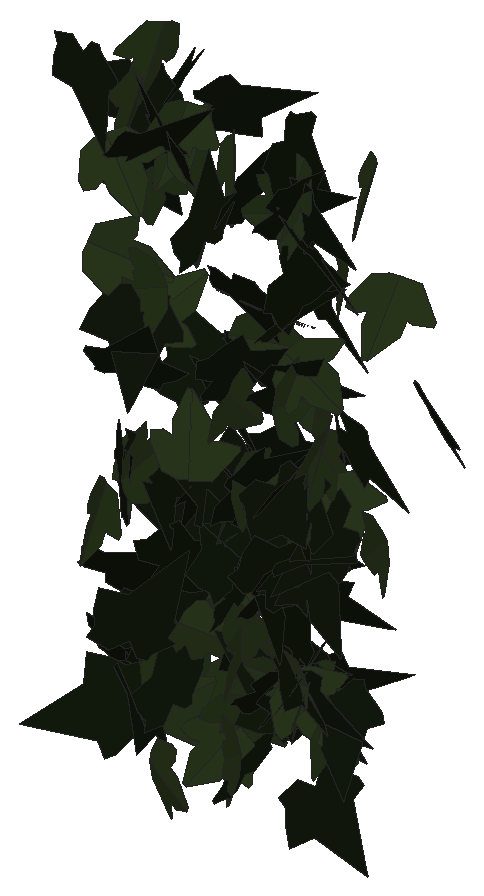
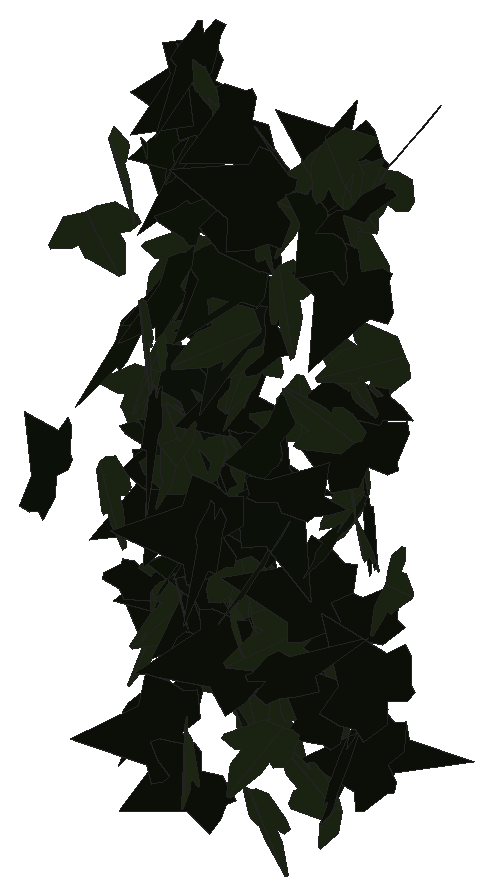
# SketchUp Ruby script. Lengths in inches.
U = 1.inch
M = Sketchup.active_model
def pt(a) = Geom::Point3d.new(a.map { |v| v * U })
def face(e, loops, mat)
  f = e.add_face(loops[0].map { |a| pt(a) })
  loops[1..].each { |l| e.add_face(l.map { |a| pt(a) }).erase! }
  f.material = f.back_material = mat if mat
  f
end
# faces: each face lists its corners as indices into pts; further lists are holes
def faces(e, pts, list, mat = nil) = list.each { |f| face(e, (f[0].is_a?(Array) ? f : [f]).map { |l| l.map { |i| pts[i] } }, mat) }
# xy, xz, yz: faces in a plane at the given z, y or x. An outline is a flat list of corners, or four numbers for a rectangle; further outlines are holes
def ring(l) = l.size == 4 ? [[l[0], l[1]], [l[2], l[1]], [l[2], l[3]], [l[0], l[3]]] : l.each_slice(2).to_a
def flat(e, list, mat, &to3) = list.each { |f| face(e, (f[0].is_a?(Array) ? f : [f]).map { |l| ring(l).map { |u, v| to3.(u, v) } }, mat) }
def xy(e, z, list, mat = nil) = flat(e, list, mat) { |x, y| [x, y, z] }
def xz(e, y, list, mat = nil) = flat(e, list, mat) { |x, z| [x, y, z] }
def yz(e, x, list, mat = nil) = flat(e, list, mat) { |y, z| [x, y, z] }
def lines(e, pts, list) = list.each { |a, b| e.add_line(pt(pts[a]), pt(pts[b])) }
# prism: a flat outline (further loops are holes) pulled along v
def prism(e, loops, v, mat = nil)
  f = face(e, loops, mat); d = Geom::Vector3d.new(v.map { |x| x * U })
  f.pushpull(f.normal.samedirection?(d) ? d.length : -d.length)
end
def box(e, o, s, mat = nil) = prism(e, [[o, [o[0] + s[0], o[1], o[2]], [o[0] + s[0], o[1] + s[1], o[2]], [o[0], o[1] + s[1], o[2]]]], [0, 0, s[2]], mat)
def at(x, y, z, deg = 0) = Geom::Transformation.translation(pt([x, y, z])) * Geom::Transformation.rotation(ORIGIN, Z_AXIS, deg.degrees)
def axes(o, x, y, z) = Geom::Transformation.new([*x, 0, *y, 0, *z, 0, *pt(o).to_a, 1])
def part(name) = M.definitions.add(name)
# library, detail: a bought-in or finely detailed component or shape, given as its bounding box
def library(name, o, s) = part(name).tap { |d| box(d.entities, o, s) }
def detail(e, o, s) = box(e.add_group.entities, o, s)
def put(e, d, t, mat = nil) = e.add_instance(d, t).tap { |i| i.material = mat if mat }
def group(e, t, mat = nil) = e.add_group.tap { |g| g.transformation = t; g.material = mat if mat }.entities
root = M.entities
M.materials.add("efeu1").color = [18, 25, 13]
M.materials.add("efeu2").color = [43, 57, 29]
c1 = part("ivyleaf_9")
p = [[1.54,2.16,1.25],[1.36,2.04,1.19],[-0.21,0.99,0.68],[-0.71,1.11,0.82],[-0.85,0.86,0.67],[-0.8,0.17,0.21],
  [-0.9,-0.01,0.1],[-0.67,-0.16,-0.02],[-0.08,-0.08,-0.05],[-0.03,-0.6,-0.4],[0.65,-0.88,-0.66],[0.83,-0.6,-0.49],
  [1.29,-0.42,-0.43],[1.8125,-0.07,-0.26],[1.21,0.44,0.15]]
faces(c1.entities,p,[[0,1,2,3,4,5,6,7,8,9,10,11,12,13,14]],"efeu1")
c2 = part("ivyleaf_10")
p = [[0,0.5,-0.03],[-0.0625,2.02,-0.43],[-0.19,2.01,-0.46],[-0.54,1.05,-0.29],[-0.52,0.625,-0.18],[-0.83,0.76,-0.28],
  [-1.16,0.64,-0.33],[-1.15,0.33,-0.24],[-0.77,-0.39,0.02],[-0.3,-0.51,0.16],[0.04,-0.48,0.23],[-0.02,2.01,-0.4375],
  [-0.06,2.01,-0.43],[0.04,-0.49,0.23],[0.67,-0.49,0.14],[1.38,0.36,-0.2],[1.375,0.51,-0.24],[0.81,0.65,-0.19],
  [0.62,0.59,-0.15],[0.6,1.09,-0.28],[0.5,1.23,-0.31]]
faces(c2.entities,p,[[0,1,2,3,4,5,6,7,8,9,10],[11,12,0,13,14,15,16,17,18,19,20]],"efeu2")
put(root,c1,axes([42.93,222.36,233.58],[0.15488,-0.47136,0.06189],[0.02451,-0.05709,-0.49613],[0.47478,0.15671,0.00543]))
put(root,c2,axes([43.24,222.41,226.64],[-0.02488,0.30941,-0.39197],[0.00458,-0.3923,-0.30996],[-0.49936,-0.01901,0.01669]))
put(root,c1,axes([42.96,222.87,225.19],[0.44169,0.18488,-0.14397],[0.13357,0.05377,0.47882],[0.19253,-0.46144,-0.00189]))
put(root,c1,axes([43.4375,223.5,232.54],[0.09096,0.30125,0.38855],[-0.03285,0.39799,-0.30088],[-0.49056,0.02921,0.09219]))
put(root,c2,axes([43.01,222.72,230.36],[0.11872,0.11072,0.47291],[0.33753,0.33126,-0.16229],[-0.34925,0.35778,0.00392]))
put(root,c1,axes([43.19,223.3,232.87],[0.01893,-0.49026,-0.09637],[-0.01328,0.09592,-0.49053],[0.49947,0.02113,-0.00939]))
put(root,c1,axes([43.28,223.01,231.71],[0.38774,0.31259,-0.04407],[-0.03007,-0.03292,-0.49801],[-0.31425,0.38885,-0.00673]))
put(root,c1,axes([43.27,223.64,223.89],[-0.00944,-0.14367,0.47882],[-0.06893,-0.47396,-0.14357],[0.49514,-0.06872,-0.01086]))
put(root,c2,axes([43.33,223.01,232.89],[0.08318,-0.37439,0.32079],[0.16253,-0.28632,-0.3763],[0.46547,0.16688,0.07406]))
put(root,c1,axes([43.01,222.79,224.13],[0.36576,-0.15936,0.30137],[0.27375,-0.12612,-0.39894],[0.20317,0.45683,-0.00501]))
put(root,c2,axes([43.44,223.34,233.63],[-0.07219,-0.46219,0.17654],[0.05138,-0.18445,-0.46189],[0.49209,-0.04854,0.07413]))
put(root,c1,axes([43.84,222.13,223.7],[-0.32895,-0.11375,0.35896],[-0.34056,-0.11349,-0.34805],[0.16066,-0.47348,-0.00281]))
put(root,c2,axes([43.85,222.74,230.08],[0.20662,-0.13869,-0.43368],[-0.37197,0.22324,-0.24861],[0.26258,0.42536,-0.01093]))
put(root,c1,axes([43.4,222.69,228.625],[0.47942,0.12712,0.06323],[-0.0611,-0.01628,0.49599],[0.12816,-0.4833,-0.00007]))
put(root,c2,axes([43.72,222.75,231.92],[-0.48355,-0.11831,0.04669],[-0.04423,-0.01567,-0.49779],[0.11925,-0.48555,0.00469]))
put(root,c1,axes([43.6,222.77,229.65],[-0.33168,-0.29939,-0.22441],[0.16944,0.14719,-0.4468],[0.33359,-0.37243,0.00381]))
put(root,c1,axes([43.97,224.05,225.63],[-0.18764,-0.4073,-0.22113],[-0.07372,-0.2093,0.44806],[-0.45755,0.20075,0.0185]))
put(root,c2,axes([43.44,223.21,229.27],[0.35959,0.00728,-0.34733],[0.33553,0.12232,0.34994],[0.09006,-0.48475,0.08308]))
put(root,c1,axes([44.03,223.76,228.27],[-0.45268,-0.21087,-0.0249],[-0.02211,-0.0115,0.49938],[-0.21118,0.45321,0.00109]))
put(root,c1,axes([43.59,222.35,227.02],[-0.04067,0.11489,0.48492],[0.10552,-0.47351,0.12104],[0.48704,0.11218,0.01426]))
put(root,c2,axes([43.62,222.55,227.51],[0.346,-0.22098,0.2854],[0.23724,-0.15873,-0.41052],[0.27204,0.41949,-0.00499]))
put(root,c2,axes([43.71,224.36,224.9375],[0.14333,0.38801,0.2809],[0.1107,0.25843,-0.41347],[-0.46605,0.18072,-0.01182]))
put(root,c2,axes([43.75,221.95,232.54],[0.35194,0.28805,0.20776],[0.14277,0.15308,-0.45408],[-0.3252,0.37894,0.0255]))
put(root,c1,axes([43.73,222.7,223.59],[0.03943,-0.33458,0.36946],[0.07022,-0.36319,-0.3364],[0.49347,0.07841,0.01835]))
put(root,c1,axes([43.8,222.72,224.47],[-0.14274,-0.05958,0.47547],[0.46927,0.08305,0.15128],[-0.09701,0.48944,0.03221]))
put(root,c2,axes([44.12,221.99,227.56],[-0.00166,-0.03063,0.49906],[-0.18943,0.4619,0.02772],[-0.46272,-0.18898,-0.01313]))
put(root,c1,axes([43.84,222.76,227.33],[0.14278,-0.44907,0.16719],[0.07176,-0.15245,-0.47076],[0.47378,0.15842,0.02092]))
put(root,c2,axes([44.32,225.4,225.125],[0.09412,-0.24121,-0.42774],[-0.14569,0.4022,-0.25886],[0.46895,0.17337,0.00542]))
put(root,c1,axes([44.3,224.9,228.29],[0.09527,-0.05421,-0.48784],[-0.39394,0.288,-0.10893],[0.29281,0.40511,0.01217]))
put(root,c2,axes([44.36,223.8,223.45],[0.41288,-0.2121,-0.18587],[-0.16028,0.09466,-0.46406],[0.23204,0.44278,0.01017]))
put(root,c2,axes([43.94,223,223.38],[0.29553,-0.11005,-0.38801],[0.37476,-0.10286,0.31461],[-0.14907,-0.47677,0.02168]))
put(root,c1,axes([44.37,222.53,232.43],[0.27121,-0.32422,0.26708],[-0.14018,0.22983,0.42134],[-0.39598,-0.30342,0.03377]))
put(root,c2,axes([44.33,222.79,232.86],[0.16871,0.41247,-0.22673],[-0.12044,-0.19501,-0.44437],[-0.45501,0.20456,0.03355]))
put(root,c1,axes([44.03,222.06,232.54],[0.27298,0.40414,-0.11023],[0.05639,0.09492,0.48766],[0.41509,-0.27868,0.00624]))
put(root,c2,axes([44.54,222.46,224.75],[-0.33088,-0.28368,0.24504],[-0.1662,-0.18194,-0.43506],[0.336,-0.36936,0.02611]))
put(root,c2,axes([44.4,223.22,231.25],[0.06924,-0.49236,-0.05277],[-0.00715,0.05229,-0.49721],[0.49513,0.06961,0.0002]))
put(root,c2,axes([44.45,222.76,232.15],[0.0746,0.2972,-0.3951],[-0.01662,0.40085,0.2984],[0.49412,-0.03139,0.06969]))
put(root,c1,axes([44.3,221.71,225.15],[-0.18705,-0.10636,0.45133],[0.43383,0.1317,0.21083],[-0.16373,0.47047,0.04301]))
put(root,c1,axes([44.3,223.59,232.74],[0.24647,0.28697,-0.32695],[0.17913,0.2755,0.37685],[0.39644,-0.3029,0.033]))
put(root,c2,axes([44.34,222.29,222.8],[-0.04784,0.06612,-0.4933],[0.36446,-0.33284,-0.07995],[-0.33895,-0.36722,-0.01635]))
put(root,c1,axes([44.33,222.38,226.01],[0.18762,0.02604,0.46273],[0.45518,0.08361,-0.18927],[-0.08724,0.49227,0.00767]))
put(root,c1,axes([44.96,221.77,224.35],[-0.45037,0.16302,-0.14348],[-0.13711,0.04272,0.47893],[0.16841,0.47074,0.00622]))
put(root,c1,axes([44.94,222.79,227.53],[-0.14688,0.43917,-0.18857],[0.04228,-0.18456,-0.46276],[-0.47606,-0.15189,0.01708]))
put(root,c1,axes([44.59,223.37,227],[0.31066,-0.36698,-0.13719],[-0.08719,0.10593,-0.48081],[0.38195,0.32266,0.00182]))
put(root,c2,axes([44.63,223.45,232.17],[0.30821,-0.23587,0.31524],[0.28349,-0.14486,-0.38555],[0.27321,0.41639,0.04444]))
put(root,c1,axes([44.58,223.125,228.7],[0.33879,-0.34494,0.12744],[0.08758,-0.09261,-0.48348],[0.35714,0.34992,-0.00233]))
put(root,c2,axes([44.93,222.34,225.24],[-0.21666,-0.10794,-0.4375],[0.39046,0.19737,-0.24205],[0.22495,-0.44654,-0.00123]))
put(root,c2,axes([45.16,221.9,228.15],[0.45099,0.21584,-0.00484],[-0.00155,0.01446,0.49979],[0.21589,-0.45078,0.01372]))
put(root,c1,axes([45.6,222.28,227.67],[-0.23885,0.16947,0.40526],[-0.3612,0.18674,-0.29097],[-0.24998,-0.43175,0.03322]))
put(root,c1,axes([45.65,221.64,231.98],[-0.41374,0.19311,-0.20378],[-0.18501,0.08545,0.45659],[0.21117,0.45322,0.00075]))
put(root,c1,axes([45.09,223.77,227.34],[0.26728,0.05029,0.41956],[0.41179,0.08036,-0.27197],[-0.09479,0.49093,0.00155]))
put(root,c1,axes([45.11,222.67,227.51],[0.09905,-0.18715,0.45295],[0.28224,-0.35601,-0.20881],[0.40066,0.29704,0.03511]))
put(root,c2,axes([45.64,222.125,223.81],[0.4238,0.02766,-0.26387],[-0.26462,0.00797,-0.42416],[-0.01926,0.49917,0.0214]))
put(root,c1,axes([45.32,223.93,223.67],[-0.029,-0.0543,-0.4962],[0.34454,0.35746,-0.05926],[0.36118,-0.34536,0.01668]))
put(root,c2,axes([45.79,223.81,228.26],[-0.00496,0.32474,-0.38016],[-0.04975,0.37797,0.32352],[0.49749,0.04103,0.02857]))
put(root,c1,axes([46.04,221.74,226.9],[-0.44598,0.05833,-0.21839],[-0.22395,-0.04836,0.44442],[0.03072,0.49423,0.06926]))
put(root,c2,axes([45.54,222.71,229.84],[0.10693,0.09472,0.47916],[0.18741,0.44501,-0.12979],[-0.45105,0.20735,0.05967]))
put(root,c2,axes([45.72,222.1875,227.2],[0.12055,-0.45222,0.17596],[-0.03408,0.17297,0.46789],[-0.48405,-0.1248,0.01087]))
put(root,c1,axes([45.83,222.32,229.79],[0.36823,0.16441,-0.2956],[-0.33811,0.16644,-0.32861],[-0.00965,0.44189,0.23375]))
put(root,c2,axes([45.76,222.47,225.41],[0.18175,-0.40168,0.23584],[0.09045,-0.21791,-0.44083],[0.45693,0.20291,-0.00654]))
put(root,c2,axes([46.04,222.125,225.8],[-0.44522,-0.07153,0.21602],[-0.21421,-0.02841,-0.4509],[0.07678,-0.49404,-0.00535]))
put(root,c2,axes([45.84,222.02,229.34],[-0.05719,-0.37095,-0.33034],[0.07093,0.32302,-0.37501],[0.49163,-0.08975,0.01568]))
put(root,c2,axes([45.92,222.17,224.31],[0.45401,0.16665,-0.12691],[-0.18354,0.17048,-0.43272],[-0.10096,0.4395,0.21598]))
put(root,c1,axes([45.56,222.73,224.95],[0.06957,0.15131,-0.47145],[0.22752,0.41307,0.16615],[0.43977,-0.23764,-0.01138]))
put(root,c1,axes([45.64,221.91,229.6],[0.19583,0.11248,0.44609],[0.36262,0.26064,-0.2249],[-0.28313,0.4116,0.02051]))
put(root,c1,axes([45.83,222.07,231.13],[0.45716,0.12402,-0.16009],[-0.16039,-0.01954,-0.47317],[-0.12362,0.48398,0.02192]))
put(root,c1,axes([45.8125,222.34,230.7],[0.46518,0.16695,-0.07574],[-0.13487,0.17176,-0.44979],[-0.12416,0.43889,0.20483]))
put(root,c1,axes([46.08,221.76,226.33],[-0.33018,0.2963,-0.23062],[-0.16987,0.156,0.44363],[0.33485,0.37131,-0.00235]))
put(root,c2,axes([46.12,221.68,223.93],[0.19613,-0.21769,-0.40515],[-0.24164,0.32599,-0.29213],[0.39133,0.3104,0.02267]))
put(root,c1,axes([45.72,222.1,226.78],[0.40914,0.23885,0.15986],[0.14097,0.07559,-0.47372],[-0.25047,0.43271,-0.00549]))
put(root,c1,axes([46,221.97,232.68],[-0.09948,0.26339,-0.4132],[-0.17573,0.3744,0.28097],[0.45741,0.20112,0.01808]))
put(root,c1,axes([46.26,221.75,223.66],[-0.06744,0.38352,0.31364],[-0.15092,0.28558,-0.38166],[-0.47188,-0.14614,0.07725]))
put(root,c2,axes([46.13,224.07,230.48],[0.24135,-0.315,-0.30418],[-0.12945,0.28048,-0.39316],[0.41832,0.26853,0.05383]))
put(root,c1,axes([45.84,223.72,224.02],[0.2859,0.08136,0.40205],[0.36165,0.18126,-0.29386],[-0.19356,0.45883,0.04479]))
put(root,c1,axes([46.4375,222.61,224.52],[-0.28602,-0.39792,-0.09924],[-0.05173,-0.08502,0.49],[-0.40684,0.29056,0.00747]))
put(root,c1,axes([46.34,223.59,228.82],[0.20002,-0.01952,-0.45783],[-0.44467,0.11243,-0.19906],[0.11071,0.48681,0.02762]))
put(root,c2,axes([46.26,221.73,228.27],[-0.10263,0.40888,0.26885],[-0.12485,0.24373,-0.41834],[-0.47316,-0.15301,0.05207]))
put(root,c1,axes([46.1875,221.62,228.16],[-0.05741,0.30934,-0.3886],[-0.12764,0.36886,0.31249],[0.48001,0.13508,0.03662]))
put(root,c1,axes([46.14,223.35,230.66],[0.40647,-0.28872,-0.03777],[-0.02862,0.02493,-0.49856],[0.28977,0.40745,0.00374]))
put(root,c1,axes([46.1875,221.92,227.43],[0.2833,0.2021,0.35902],[0.27188,0.23566,-0.3472],[-0.30955,0.39194,0.02363]))
put(root,c2,axes([46.4,222.79,227.47],[-0.24498,-0.42378,0.10196],[0.06736,0.07875,0.48914],[-0.43064,0.2534,0.01851]))
put(root,c2,axes([46.8,222,232.625],[0.2109,-0.08366,-0.44556],[-0.40421,0.18781,-0.2266],[0.20527,0.45577,0.01158]))
put(root,c1,axes([46.3125,222.13,226.63],[0.15814,-0.4299,0.20045],[0.05997,-0.19148,-0.45797],[0.47053,0.16889,-0.009]))
put(root,c1,axes([46.5625,221.68,226.62],[0.13834,0.31097,0.36627],[0.11496,0.34866,-0.33944],[-0.46653,0.17813,0.02497]))
put(root,c1,axes([47,221.94,227.26],[-0.24281,0.06198,0.43267],[-0.41482,0.12326,-0.25046],[-0.1377,-0.48059,-0.00844]))
put(root,c1,axes([46.54,221.73,225.0625],[0.30171,0.31682,0.24207],[0.12744,0.211,-0.43501],[-0.3778,0.32419,0.04657]))
put(root,c2,axes([47.08,221.77,225.37],[0.09158,-0.02031,-0.49112],[-0.45071,0.19588,-0.09215],[0.19615,0.45959,0.01757]))
put(root,c1,axes([46.9375,221.92,228.48],[-0.0879,0.49026,0.04384],[-0.00876,0.04297,-0.49807],[-0.49213,-0.08833,0.00103]))
put(root,c1,axes([47.14,221.9,227.68],[-0.07577,0.0455,-0.49213],[-0.49384,-0.02672,0.07356],[-0.0196,0.49721,0.04899]))
put(root,c1,axes([46.8,222.01,233.7],[0.14336,-0.17868,-0.44444],[-0.27935,0.34567,-0.22907],[0.38912,0.31398,-0.00072]))
put(root,c2,axes([46.85,222.11,228.07],[0.45054,-0.18871,-0.10677],[-0.09639,0.04622,-0.48844],[0.19421,0.46071,0.00527]))
put(root,c2,axes([46.93,222.13,228.02],[-0.27698,-0.41504,-0.03201],[0.01977,0.02529,-0.49897],[0.4158,-0.27767,0.00241]))
put(root,c1,axes([47.17,221.79,225.86],[0.01942,-0.02132,0.49917],[-0.21026,0.4528,0.02752],[-0.45322,-0.21098,0.00862]))
put(root,c1,axes([46.86,222.21,227.1],[0.38097,0.31712,-0.06554],[-0.04295,-0.05082,-0.49555],[-0.32096,0.38321,-0.01148]))
put(root,c1,axes([46.9375,221.82,231.75],[0.09863,0.03026,-0.48924],[-0.267,0.42183,-0.02773],[0.41107,0.26673,0.09937]))
put(root,c2,axes([46.91,222.06,233.22],[0.45088,-0.21605,-0.00571],[-0.00491,0.00296,-0.49997],[0.21607,0.4509,0.00055]))
put(root,c1,axes([46.73,221.77,229.92],[0.33483,0.23697,0.2859],[0.23328,0.16529,-0.4102],[-0.28892,0.40808,0.00013]))
put(root,c2,axes([46.98,223.6,232.53],[0.29352,-0.40478,0.00094],[0.00053,-0.00078,-0.5],[0.40478,0.29352,-0.00003]))
put(root,c1,axes([47,221.61,225.0625],[-0.21907,0.42015,-0.15964],[-0.07245,0.14225,0.47383],[0.44358,0.23073,-0.00144]))
put(root,c1,axes([46.78,221.63,226.84],[-0.04848,-0.04635,0.49548],[0.46756,0.16623,0.06129],[-0.1704,0.46928,0.02722]))
put(root,c2,axes([47.06,222.12,225.15],[0.25386,-0.42651,-0.06035],[-0.03104,0.05176,-0.49634],[0.42964,0.25575,-0.0002]))
put(root,c2,axes([47.14,221.53,229.84],[-0.06428,0.12284,0.48039],[-0.21788,0.42815,-0.13863],[-0.44542,-0.22716,-0.00152]))
put(root,c1,axes([46.92,221.64,232.82],[0.21717,0.29873,0.33704],[0.20374,0.26854,-0.36929],[-0.40166,0.29773,-0.00509]))
put(root,c2,axes([46.94,222.1,224.99],[-0.14154,-0.21402,-0.42914],[0.24019,0.35564,-0.25658],[0.41506,-0.27878,0.00213]))
put(root,c1,axes([46.73,222.17,230.88],[0.17196,-0.45567,0.11312],[0.4602,0.18744,0.05548],[-0.09297,0.08504,0.48387]))
put(root,c1,axes([46.84,221.79,228.33],[-0.0502,-0.18149,-0.46319],[0.28995,0.36762,-0.17547],[0.40424,-0.28622,0.06834]))
put(root,c1,axes([46.84,222.16,232.27],[0.37821,-0.30523,0.11746],[0.09959,-0.06356,-0.48584],[0.31152,0.39089,0.01271]))
put(root,c1,axes([47.02,222.01,225.6],[0.25246,-0.37459,-0.21435],[-0.12356,0.1752,-0.4517],[0.41352,0.28104,-0.00411]))
put(root,c2,axes([47.0625,221.93,230.3],[0.12237,0.37203,0.31083],[0.07541,0.30207,-0.39124],[-0.47889,0.14263,0.01782]))
put(root,c1,axes([46.85,222.05,232.82],[0.0981,0.0249,-0.48965],[0.46866,0.14189,0.10111],[0.14399,-0.4788,0.0045]))
put(root,c2,axes([47.28,222.17,229.09],[0.15015,-0.47686,-0.00759],[-0.00166,0.00743,-0.49994],[0.47692,0.15016,0.00065]))
put(root,c1,axes([46.89,221.87,225.13],[0.06453,0.04688,-0.4936],[0.37747,0.3181,0.07957],[0.32148,-0.3829,0.00566]))
put(root,c1,axes([46.95,225,228.21],[0.32888,-0.06855,-0.37032],[0.36663,-0.05418,0.33563],[-0.08614,-0.49231,0.01462]))
put(root,c1,axes([47.04,222.05,226.63],[0.4315,0.14461,0.2071],[0.19704,0.06379,-0.45509],[-0.15804,0.47436,-0.00194]))
put(root,c2,axes([47.52,223.13,227.11],[0.29328,-0.16032,-0.37186],[-0.23646,0.30494,-0.31796],[0.32874,0.36237,0.10305]))
put(root,c2,axes([47.2,221.75,225.25],[0.17713,0.40009,0.24199],[0.10082,0.22,-0.43753],[-0.45658,0.20379,-0.00273]))
put(root,c1,axes([47.23,222.15,223.54],[0.1013,-0.35054,-0.34185],[-0.06659,0.33598,-0.36425],[0.48508,0.11932,0.02139]))
put(root,c2,axes([47.34,222.15,228.84],[0.11419,-0.41918,-0.24749],[0.14044,0.27176,-0.3955],[0.46609,0.02081,0.1798]))
put(root,c1,axes([47.18,221.95,227.28],[-0.17365,-0.18789,-0.42958],[0.37838,0.21438,-0.24672],[0.2769,-0.41077,0.06773]))
put(root,c2,axes([47.38,222.14,224.59],[0.11371,-0.40086,-0.27637],[0.13973,0.29873,-0.37581],[0.46642,0.00823,0.17996]))
put(root,c1,axes([47.74,222.01,227.92],[-0.4972,0.04999,-0.01701],[0.01687,-0.0023,-0.49971],[-0.05004,-0.49749,0.0006]))
put(root,c1,axes([47.18,222.125,227.36],[0.04899,-0.49429,0.05727],[0.48904,0.03721,-0.09725],[0.09188,0.06554,0.4871]))
put(root,c2,axes([47.43,222.26,228.26],[0.36748,0.31277,0.13088],[0.0991,0.0855,-0.48256],[-0.32424,0.38061,0.00085]))
put(root,c1,axes([47.56,222.19,225.14],[-0.30555,-0.24652,-0.30962],[0.22793,0.21017,-0.39227],[0.32356,-0.38086,-0.01606]))
put(root,c2,axes([47.6875,223.25,231.09],[0.36218,0.30073,-0.16847],[-0.13648,-0.09929,-0.47065],[-0.31654,0.38691,0.01016]))
put(root,c1,axes([47.57,222.45,229.14],[0.40155,-0.21643,-0.20473],[-0.14774,0.15371,-0.45227],[0.25871,0.42371,0.05949]))
